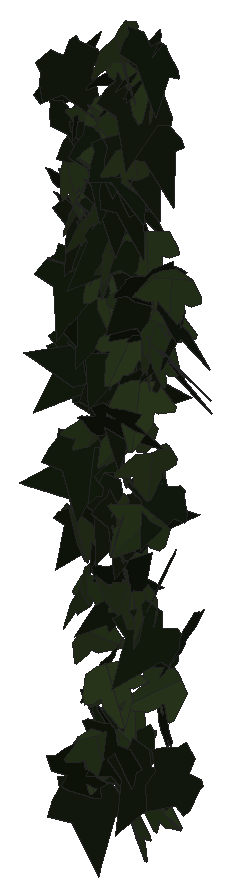
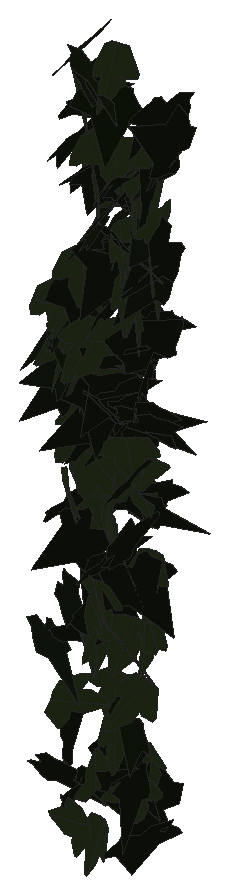
# SketchUp Ruby script. Lengths in inches.
U = 1.inch
M = Sketchup.active_model
def pt(a) = Geom::Point3d.new(a.map { |v| v * U })
def face(e, loops, mat)
  f = e.add_face(loops[0].map { |a| pt(a) })
  loops[1..].each { |l| e.add_face(l.map { |a| pt(a) }).erase! }
  f.material = f.back_material = mat if mat
  f
end
# faces: each face lists its corners as indices into pts; further lists are holes
def faces(e, pts, list, mat = nil) = list.each { |f| face(e, (f[0].is_a?(Array) ? f : [f]).map { |l| l.map { |i| pts[i] } }, mat) }
# xy, xz, yz: faces in a plane at the given z, y or x. An outline is a flat list of corners, or four numbers for a rectangle; further outlines are holes
def ring(l) = l.size == 4 ? [[l[0], l[1]], [l[2], l[1]], [l[2], l[3]], [l[0], l[3]]] : l.each_slice(2).to_a
def flat(e, list, mat, &to3) = list.each { |f| face(e, (f[0].is_a?(Array) ? f : [f]).map { |l| ring(l).map { |u, v| to3.(u, v) } }, mat) }
def xy(e, z, list, mat = nil) = flat(e, list, mat) { |x, y| [x, y, z] }
def xz(e, y, list, mat = nil) = flat(e, list, mat) { |x, z| [x, y, z] }
def yz(e, x, list, mat = nil) = flat(e, list, mat) { |y, z| [x, y, z] }
def lines(e, pts, list) = list.each { |a, b| e.add_line(pt(pts[a]), pt(pts[b])) }
# prism: a flat outline (further loops are holes) pulled along v
def prism(e, loops, v, mat = nil)
  f = face(e, loops, mat); d = Geom::Vector3d.new(v.map { |x| x * U })
  f.pushpull(f.normal.samedirection?(d) ? d.length : -d.length)
end
def box(e, o, s, mat = nil) = prism(e, [[o, [o[0] + s[0], o[1], o[2]], [o[0] + s[0], o[1] + s[1], o[2]], [o[0], o[1] + s[1], o[2]]]], [0, 0, s[2]], mat)
def at(x, y, z, deg = 0) = Geom::Transformation.translation(pt([x, y, z])) * Geom::Transformation.rotation(ORIGIN, Z_AXIS, deg.degrees)
def axes(o, x, y, z) = Geom::Transformation.new([*x, 0, *y, 0, *z, 0, *pt(o).to_a, 1])
def part(name) = M.definitions.add(name)
# library, detail: a bought-in or finely detailed component or shape, given as its bounding box
def library(name, o, s) = part(name).tap { |d| box(d.entities, o, s) }
def detail(e, o, s) = box(e.add_group.entities, o, s)
def put(e, d, t, mat = nil) = e.add_instance(d, t).tap { |i| i.material = mat if mat }
def group(e, t, mat = nil) = e.add_group.tap { |g| g.transformation = t; g.material = mat if mat }.entities
root = M.entities
M.materials.add("efeu1").color = [18, 25, 13]
M.materials.add("efeu2").color = [43, 57, 29]
c1 = part("ivyleaf_9")
p = [[1.54,2.16,1.25],[1.36,2.04,1.19],[-0.21,0.99,0.68],[-0.71,1.11,0.82],[-0.85,0.86,0.67],[-0.8,0.17,0.21],
  [-0.9,-0.01,0.1],[-0.67,-0.16,-0.02],[-0.08,-0.08,-0.05],[-0.03,-0.6,-0.4],[0.65,-0.88,-0.66],[0.83,-0.6,-0.49],
  [1.29,-0.42,-0.43],[1.8125,-0.07,-0.26],[1.21,0.44,0.15]]
faces(c1.entities,p,[[0,1,2,3,4,5,6,7,8,9,10,11,12,13,14]],"efeu1")
c2 = part("ivyleaf_10")
p = [[0,0.5,-0.03],[-0.0625,2.02,-0.43],[-0.19,2.01,-0.46],[-0.54,1.05,-0.29],[-0.52,0.625,-0.18],[-0.83,0.76,-0.28],
  [-1.16,0.64,-0.33],[-1.15,0.33,-0.24],[-0.77,-0.39,0.02],[-0.3,-0.51,0.16],[0.04,-0.48,0.23],[-0.02,2.01,-0.4375],
  [-0.06,2.01,-0.43],[0.04,-0.49,0.23],[0.67,-0.49,0.14],[1.38,0.36,-0.2],[1.375,0.51,-0.24],[0.81,0.65,-0.19],
  [0.62,0.59,-0.15],[0.6,1.09,-0.28],[0.5,1.23,-0.31]]
faces(c2.entities,p,[[0,1,2,3,4,5,6,7,8,9,10],[11,12,0,13,14,15,16,17,18,19,20]],"efeu2")
put(root,c1,axes([555.37,131.1,236.45],[0.02689,-0.13384,0.95916],[0.62063,0.73899,0.08572],[-0.74346,0.61205,0.10625]))
put(root,c1,axes([555.43,131.6,232.75],[0.95601,0.10212,-0.10441],[-0.1051,0.00093,-0.96137],[-0.10142,0.96169,0.01202]))
put(root,c2,axes([555.83,131.82,231.69],[0.41811,-0.87537,-0.0637],[0.06127,0.0995,-0.96514],[0.87555,0.41107,0.09797]))
put(root,c1,axes([556.1875,132.05,225.11],[-0.8463,-0.33405,0.13391],[-0.10601,-0.09561,-0.9085],[0.34393,-0.85148,0.04948]))
put(root,c1,axes([556.11,132.44,225.83],[-0.7996,-0.47085,-0.07469],[0.06122,0.04323,-0.92791],[0.47279,-0.80191,-0.00616]))
put(root,c1,axes([555.62,131.73,231.7],[0.94441,0.04045,-0.16656],[-0.16916,0.0696,-0.94224],[-0.02763,0.95645,0.07561]))
put(root,c1,axes([556.18,131.64,234.32],[0.02952,-0.38642,0.96852],[0.17134,0.95754,0.37682],[-1.02859,0.14841,0.09056]))
put(root,c1,axes([556.8,132.03,224.96],[-0.44942,0.0005,0.89544],[-0.89541,0.00788,-0.44941],[-0.00727,-1.00186,-0.00308]))
put(root,c1,axes([556.28,132.41,210.52],[0.68966,0.055,-0.739],[-0.74058,0.01515,-0.69],[-0.02643,1.01071,0.05055]))
put(root,c2,axes([556.1,131.22,233.5],[-0.08963,0.96019,0.05758],[-0.04433,0.05364,-0.96357],[-0.96089,-0.09204,0.03908]))
put(root,c1,axes([556.53,132.11,218.81],[0.18482,0.5254,-0.84591],[-0.2453,-0.80982,-0.55658],[-0.9651,0.30645,-0.02053]))
put(root,c2,axes([556.34,131.32,218.85],[-0.89072,0.24427,0.11586],[-0.11013,0.0365,-0.92359],[-0.24691,-0.89748,-0.00603]))
put(root,c1,axes([556.92,131.26,220.96],[-0.73932,0.08568,0.56516],[-0.56781,-0.00366,-0.74224],[-0.06584,-0.93058,0.05495]))
put(root,c1,axes([555.93,131.05,238.15],[0.17485,-0.71635,-0.68512],[-0.1145,0.67644,-0.7365],[0.9846,0.20588,0.03602]))
put(root,c1,axes([556.24,131.6,229.28],[-0.66043,-0.65762,-0.18862],[0.14763,0.11899,-0.9318],[0.66801,-0.67645,0.01946]))
put(root,c1,axes([555.76,132.01,228.4],[1.03081,0.17194,0.04386],[-0.04432,-0.00091,1.04503],[0.17182,-1.03174,0.00639]))
put(root,c1,axes([555.95,133.19,223.28],[0.14447,-0.90416,0.10259],[0.01665,-0.10123,-0.91563],[0.90981,0.14543,0.00047]))
put(root,c2,axes([556.2,132.81,224.5],[0.80714,0.45763,-0.05627],[-0.0491,-0.0275,-0.92785],[-0.45846,0.80863,0.00029]))
put(root,c1,axes([555.76,131.59,235.57],[0.36085,-0.89036,0.19543],[0.20608,-0.12506,-0.95029],[0.88796,0.39086,0.14113]))
put(root,c1,axes([556.51,133.11,220.03],[-0.22171,-0.14264,0.88694],[-0.4483,-0.77409,-0.23656],[0.77848,-0.4864,0.11637]))
put(root,c1,axes([556.67,131.01,232.82],[0.00508,0.63079,0.83793],[0.01187,0.83785,-0.6308],[-1.04875,0.01254,-0.00308]))
put(root,c2,axes([556.55,131.09,216.12],[0.07164,-0.73017,-0.69798],[-0.07508,0.69395,-0.73366],[1.00732,0.10365,-0.00504]))
put(root,c2,axes([556.26,132.09,213.88],[-0.25192,-0.54666,-0.73995],[0.35186,0.65161,-0.60119],[0.85003,-0.43174,0.02956]))
put(root,c1,axes([556.26,132.14,231.06],[-0.25038,-0.80938,0.46528],[0.00867,-0.48372,-0.83679],[0.93354,-0.21258,0.13256]))
put(root,c1,axes([556.16,132.15,226.375],[0.33959,-0.73444,-0.50214],[0.51009,-0.27964,0.75397],[-0.72894,-0.53784,0.29368]))
put(root,c1,axes([556.85,131.86,212.31],[-0.15047,0.76761,0.52063],[-0.08965,0.51293,-0.78217],[-0.92317,-0.17493,-0.00891]))
put(root,c2,axes([556.51,131.97,229.97],[0.59829,-0.73894,-0.21917],[-0.00107,0.27665,-0.93568],[0.77076,0.57398,0.16883]))
put(root,c2,axes([556.72,131.83,222.77],[-0.31262,-0.83811,0.26236],[-0.09271,-0.24543,-0.89451],[0.8733,-0.32608,-0.00105]))
put(root,c2,axes([556.61,132.43,230.98],[0.00044,-0.93504,-0.1991],[0.04483,0.1989,-0.93401],[0.95495,-0.00891,0.04394]))
put(root,c1,axes([556.45,131.5625,221.89],[-0.36618,-0.84517,-0.20789],[0.08134,0.19133,-0.92108],[0.86655,-0.37511,-0.00139]))
put(root,c2,axes([556.66,131.73,233.89],[0.34195,-0.90255,-0.20089],[-0.0009,0.21386,-0.96236],[0.92463,0.33399,0.07335]))
put(root,c1,axes([556.43,132.61,219.1],[-0.5592,0.00614,-0.72735],[0.71672,-0.1518,-0.55231],[-0.12404,-0.90482,0.08772]))
put(root,c2,axes([557.1,131.57,235.76],[-0.87232,-0.29938,0.29897],[-0.27884,-0.10846,-0.9222],[0.31821,-0.91574,0.01148]))
put(root,c1,axes([556.77,132.34,227.85],[-0.58465,-0.7611,-0.0035],[0.09169,-0.06604,-0.95306],[0.75557,-0.58092,0.11294]))
put(root,c1,axes([556.52,131.73,207.46],[-0.12604,-1.01416,-0.28006],[0.09635,0.26975,-1.02019],[1.04769,-0.14681,0.06013]))
put(root,c2,axes([556.74,131.82,209.4],[0.65969,0.57269,-0.04042],[-0.03054,-0.02648,-0.8736],[-0.57331,0.6604,0.00002]))
put(root,c2,axes([556.87,131.97,216.18],[-0.82623,-0.33268,-0.21949],[0.19686,0.09862,-0.89052],[0.34655,-0.84918,-0.01743]))
put(root,c1,axes([557.72,131.77,232.06],[-0.54638,0.47653,0.63127],[-0.52747,0.35218,-0.7224],[-0.58937,-0.75697,0.0613]))
put(root,c2,axes([557,131.8125,231.49],[0.24326,-0.88016,-0.33975],[0.05396,0.36327,-0.90244],[0.94191,0.2065,0.13944]))
put(root,c1,axes([556.27,130.92,208.41],[0.34963,0.01544,0.92468],[0.92348,0.04718,-0.34996],[-0.04959,0.98744,0.00227]))
put(root,c2,axes([557.15,130.87,231.93],[0.03796,-0.90385,-0.38317],[0.01737,0.38401,-0.90412],[0.98156,0.02816,0.03082]))
put(root,c1,axes([557.13,132.35,226.26],[-0.41627,-0.8496,0.05665],[-0.01456,-0.05594,-0.94602],[0.85136,-0.41636,0.01152]))
put(root,c2,axes([557.3125,132.17,212.13],[-0.10485,-0.88455,-0.2076],[0.0422,0.20401,-0.89057],[0.9076,-0.11168,0.01742]))
put(root,c1,axes([557,131.64,234.95],[-0.19642,-0.93581,-0.22969],[0.06542,0.22092,-0.95603],[0.96137,-0.20623,0.01813]))
put(root,c1,axes([557.72,131.97,215.96],[-0.84974,0.41026,-0.04875],[0.04345,-0.02213,-0.94359],[-0.41085,-0.85085,0.00103]))
put(root,c2,axes([557.13,132.03,228.97],[0.40989,0.86251,-0.02569],[-0.01207,-0.02271,-0.95495],[-0.8628,0.41007,0.00116]))
put(root,c2,axes([557.4375,131.65,232.45],[0.05668,-0.97046,-0.11411],[-0.02143,0.11304,-0.972],[0.97691,0.05879,-0.0147]))
put(root,c1,axes([557.27,132.65,219.58],[-0.36141,-0.85485,0.15106],[-0.03543,-0.14896,-0.92778],[0.86738,-0.36228,0.02504]))
put(root,c2,axes([557.42,132.08,236.26],[0.67745,0.69462,-0.04585],[-0.13272,0.06607,-0.95997],[-0.68336,0.67578,0.14099]))
put(root,c2,axes([557.58,130.92,210.1875],[-0.58883,-0.73215,-0.18983],[0.12308,0.14462,-0.93954],[0.74628,-0.60154,0.00517]))
put(root,c1,axes([557.83,132.06,231.84],[-0.80782,-0.49938,0.1584],[-0.1093,-0.12406,-0.94853],[0.51237,-0.8138,0.0474]))
put(root,c1,axes([557.47,131.75,226.53],[0.52794,0.75081,0.22186],[0.09468,0.20439,-0.91702],[-0.77716,0.53494,0.03899]))
put(root,c2,axes([557.1,130.92,209.91],[-0.57511,-0.04177,-0.72546],[0.71937,0.09804,-0.57593],[0.10271,-0.92056,-0.02842]))
put(root,c1,axes([557.24,132.37,224.3],[0.08937,-1.07301,0.08296],[0.01113,-0.08232,-1.07672],[1.07616,0.08996,0.00425]))
put(root,c1,axes([558.27,132.12,209.13],[-0.84316,-0.36222,-0.24054],[-0.20429,-0.13328,0.91678],[-0.38383,0.86662,0.04045]))
put(root,c1,axes([557.78,132.25,226.32],[0.39759,0.83244,-0.21397],[-0.12073,-0.17933,-0.922],[-0.85097,0.41437,0.03083]))
put(root,c1,axes([558.28,131.01,210.27],[0.21497,0.13655,-1.04401],[-0.91033,-0.51132,-0.25432],[-0.52907,0.93527,0.01339]))
put(root,c1,axes([557.42,131.68,234.67],[-0.10943,-0.97813,0.07502],[-0.00037,-0.07545,-0.9842],[0.981,-0.10914,0.008]))
put(root,c1,axes([557.64,131.6875,231.49],[0.4869,0.817,0.23185],[0.07638,0.22405,-0.94989],[-0.84582,0.49055,0.04769]))
put(root,c2,axes([557.63,132.83,218.04],[0.86608,-0.24935,-0.03911],[-0.03626,0.0154,-0.90125],[0.24978,0.86682,0.00476]))
put(root,c1,axes([557.98,131.55,238.1],[0.23705,0.94658,0.0071],[-0.15645,0.0464,-0.96209],[-0.93358,0.23257,0.16303]))
put(root,c2,axes([558.13,132.36,222.94],[-0.44824,-0.6664,0.65634],[-0.33743,-0.56359,-0.80268],[0.87235,-0.56041,0.02677]))
put(root,c1,axes([557.6,132.69,219.03],[-0.13623,-0.89265,0.25627],[0.02598,-0.26258,-0.9008],[0.92835,-0.12364,0.06282]))
put(root,c2,axes([557.74,132.94,217.34],[0.15481,-0.78586,0.41306],[0.23073,-0.36928,-0.78902],[0.85729,0.24129,0.13777]))
put(root,c2,axes([557.43,130.61,234.48],[-0.59104,-0.30552,-0.7503],[0.69421,0.28772,-0.66401],[0.41757,-0.91076,0.04193]))
put(root,c2,axes([557.75,132.65,215.86],[-0.04742,-0.87433,0.09197],[0.31861,-0.10293,-0.81428],[0.81939,-0.01058,0.32195]))
put(root,c2,axes([557.99,132.21,226.62],[0.65257,0.57554,-0.37706],[-0.29475,-0.23575,-0.86996],[-0.62173,0.71586,0.01666]))
put(root,c2,axes([558.29,131.42,221.94],[-0.64742,0.41756,0.57915],[-0.47062,0.33834,-0.77004],[-0.53692,-0.80005,-0.02339]))
put(root,c2,axes([558.01,132.43,209.49],[0.10325,0.88613,-0.27267],[0.03354,0.27061,0.89213],[0.92653,-0.10855,-0.00191]))
put(root,c1,axes([558.19,131.49,231.25],[-0.72877,-0.55795,0.26405],[-0.13803,-0.25088,-0.91111],[0.60164,-0.7334,0.1108]))
put(root,c2,axes([558.07,131.36,230.68],[0.24632,-0.93465,0.15357],[0.01468,-0.15489,-0.96624],[0.94707,0.2455,-0.02496]))
put(root,c1,axes([557.53,131.98,216.42],[0.85104,0.44597,-0.04084],[0.02214,0.0457,0.96034],[0.44729,-0.8508,0.03017]))
put(root,c2,axes([557.94,131.54,218.59],[-0.51756,0.7016,-0.18904],[0.1273,-0.14095,-0.87165],[-0.71539,-0.53267,-0.01834]))
put(root,c2,axes([558.15,131.22,239.49],[-0.11061,-0.90914,-0.53316],[0.11931,0.52184,-0.91459],[1.04717,-0.15549,0.04789]))
put(root,c1,axes([558.3,132.72,225.72],[-0.88539,-0.12323,-0.29911],[0.2959,0.04381,-0.89392],[0.13076,-0.93352,-0.00246]))
put(root,c1,axes([557.69,131.54,232.85],[0.12965,-0.87065,0.39052],[0.15985,-0.36873,-0.87512],[0.94073,0.18264,0.09488]))
put(root,c2,axes([558.18,130.85,231.21],[0.31565,-0.74545,-0.55087],[0.11202,0.60835,-0.75905],[0.92011,0.18167,0.28139]))
put(root,c2,axes([558.2,131.54,219.82],[0.56772,-0.73605,0.04453],[0.02406,-0.03767,-0.92955],[0.73701,0.56822,-0.00395]))
put(root,c2,axes([557.99,132.39,228.37],[-0.74867,-0.53494,-0.57908],[0.49053,0.30908,-0.9197],[0.61715,-0.8946,0.02852]))
put(root,c1,axes([557.91,132.1,233.21],[0.72524,-0.56517,-0.29595],[-0.16968,0.26106,-0.91434],[0.61499,0.73851,0.09673]))
put(root,c2,axes([558.05,130.89,213.11],[0.73225,0.52314,0.32536],[0.25631,0.20087,-0.89982],[-0.56022,0.77569,0.01359]))
put(root,c1,axes([557.91,130.55,224.08],[0.91751,0.30543,0.28421],[0.26659,0.09896,-0.96697],[-0.32093,0.95541,0.0093]))
put(root,c2,axes([558.4,131.86,207.11],[-0.80346,0.49539,-0.05629],[0.04677,-0.03139,-0.9439],[-0.49637,-0.80482,0.00217]))
put(root,c1,axes([558.3,132.33,228.42],[-0.13047,-0.58301,0.7306],[-0.14285,-0.71658,-0.59733],[0.92372,-0.19316,0.01081]))
put(root,c1,axes([558.03,131.73,233.32],[0.34554,-0.91916,-0.07585],[-0.01332,0.07602,-0.98186],[0.92219,0.3455,0.01424]))
put(root,c1,axes([558.24,131.68,224.67],[0.11434,0.20457,-0.93331],[-0.13286,0.93424,0.18849],[0.94618,0.10647,0.13925]))
put(root,c1,axes([558.27,131.49,235.01],[-0.06439,-0.84508,-0.50202],[0.02345,0.50163,-0.84743],[0.98266,-0.06735,-0.01267]))
put(root,c1,axes([559.15,131.32,238.83],[-0.33757,0.84818,0.36437],[-0.29833,0.26691,-0.89771],[-0.8736,-0.4189,0.16577]))
put(root,c2,axes([558.57,131.88,234.6875],[0.56151,-0.7898,-0.14836],[0.0113,0.18873,-0.96195],[0.80353,0.54926,0.1172]))
put(root,c2,axes([558.89,130.91,238.84],[-0.53194,0.61068,0.57282],[-0.41468,0.39743,-0.80877],[-0.72739,-0.67316,0.04216]))
put(root,c2,axes([558.37,131.02,216.04],[-0.82267,0.13145,0.47615],[0.47289,-0.05766,0.83296],[0.14271,0.94878,-0.01535]))
put(root,c2,axes([559.08,131.01,238.18],[0.72026,-0.18086,-0.65603],[-0.62482,0.2027,-0.74188],[0.26961,0.95293,0.03329]))
put(root,c2,axes([558.92,132.23,215.78],[0.62835,-0.57421,-0.46324],[-0.32419,0.33168,-0.85089],[0.66273,0.70668,0.02297]))
put(root,c2,axes([558.75,132.3,226.66],[-0.30229,0.89132,-0.01357],[-0.1077,-0.05074,-0.93373],[-0.8849,-0.29831,0.11828]))
put(root,c1,axes([559.22,131.54,238.625],[-0.7738,0.53138,-0.28784],[0.15785,-0.27369,-0.9296],[-0.58336,-0.77891,0.13027]))
put(root,c2,axes([558.9375,132.09,231.09],[-0.72722,-0.64057,0.00499],[0.10096,-0.12207,-0.95609],[0.63258,-0.71692,0.15833]))
put(root,c2,axes([558.8125,131.68,224.81],[0.58903,0.82635,-0.14893],[-0.09727,-0.11354,-1.01471],[-0.83401,0.59686,0.01316]))
put(root,c1,axes([559.17,131.68,229.84],[0.21098,0.90775,-0.17965],[-0.05123,-0.17252,-0.93189],[-0.92394,0.21685,0.01064]))
put(root,c2,axes([559.56,131.23,219.94],[-0.65043,-0.42498,0.68169],[-0.53932,-0.41904,-0.77582],[0.59535,-0.8439,0.04195]))
put(root,c1,axes([558.57,131.77,235.05],[0.14634,-0.94407,-0.24076],[0.17101,0.26457,-0.93349],[0.95916,0.09687,0.20317]))
put(root,c1,axes([558.95,132.14,209.03],[-0.26216,-0.9,0.43293],[-0.12078,-0.41575,-0.9374],[0.99138,-0.28864,0.00028]))
put(root,c1,axes([558.97,131.75,219.52],[-0.11012,0.32552,-0.88746],[-0.22217,0.85953,0.34284],[0.9188,0.24685,-0.02347]))
put(root,c2,axes([559.55,132.55,212.57],[0.24731,0.21547,-0.88754],[-0.62053,-0.63504,-0.32708],[-0.67015,0.66754,-0.02467]))
put(root,c2,axes([559.22,130.92,235.36],[-0.3923,-0.87903,-0.171],[0.15153,0.11884,-0.95852],[0.8826,-0.41112,0.08855]))
put(root,c1,axes([559.4,132.54,217.27],[-0.57914,0.47345,-0.48352],[0.38221,-0.29634,-0.74796],[-0.55845,-0.69381,-0.01048]))
put(root,c2,axes([558.85,131.93,215.65],[-0.03544,-0.17673,0.90925],[0.59532,-0.70145,-0.11314],[0.70963,0.57963,0.14032]))
put(root,c1,axes([559.63,132.28,210.74],[0.07146,-0.34285,0.88112],[-0.26362,0.84136,0.34876],[-0.90797,-0.27126,-0.03191]))
put(root,c2,axes([559.05,132.85,221.77],[0.64269,-0.56124,0.32236],[0.24268,-0.21217,-0.85325],[0.6,0.68699,-0.00018]))
put(root,c1,axes([559.17,131.46,237.57],[-0.30438,-0.95298,0.01238],[0.01831,-0.01885,-1.00014],[0.95289,-0.30405,0.02318]))
put(root,c2,axes([558.73,132.54,207.59],[-0.23692,0.06611,-0.90975],[0.79716,-0.44184,-0.23971],[-0.44334,-0.82979,0.05516]))
put(root,c2,axes([559.46,132.12,229.62],[-0.75634,-0.51273,-0.26013],[0.20416,0.16231,-0.91355],[0.53747,-0.78318,-0.01903]))
put(root,c2,axes([559.67,131.51,238.14],[0.6064,-0.69178,-0.3586],[-0.19172,0.30796,-0.9183],[0.75525,0.63362,0.05481]))
put(root,c1,axes([559.7,131.78,215.29],[-0.63534,-0.68062,0.22577],[-0.1616,-0.15798,-0.93102],[0.69864,-0.65549,-0.01003]))
put(root,c1,axes([560,132.22,227.34],[-0.73613,0.55613,-0.23962],[0.18643,-0.15073,-0.92256],[-0.57615,-0.75933,0.00763]))
put(root,c1,axes([559.5,132.42,220.82],[-0.26124,-0.82563,0.29254],[-0.03869,-0.2941,-0.86458],[0.87507,-0.25948,0.04911]))
put(root,c1,axes([559.24,132.52,226.15],[0.91229,-0.24716,-0.00393],[-0.00379,0.00103,-0.94518],[0.24717,0.9123,0]))
put(root,c2,axes([559.9,131.04,222.76],[-0.46242,-0.84291,-0.01694],[-0.00308,0.02101,-0.96134],[0.84308,-0.46226,-0.01281]))
put(root,c2,axes([559.5625,131.94,228.05],[-0.21561,-0.56493,-0.76325],[0.41673,0.64699,-0.5966],[0.85325,-0.45875,0.09851]))
put(root,c2,axes([559.9,131.48,227.18],[-0.34796,0.69214,0.66915],[-0.26771,0.61389,-0.77419],[-0.92474,-0.43816,-0.02766]))
put(root,c2,axes([559.93,132.24,229.41],[-0.72918,-0.6166,0.08605],[0.02007,-0.15573,-0.94586],[0.62225,-0.71753,0.13134]))
put(root,c1,axes([559.46,131.71,236.04],[0.26061,-0.92629,-0.17661],[-0.01183,0.18,-0.96155],[0.9429,0.25827,0.03674]))
put(root,c1,axes([559.43,131.65,239.51],[0.09686,-0.94135,0.27937],[0.15463,-0.26259,-0.93845],[0.96967,0.13591,0.12175]))
put(root,c1,axes([559.21,132.3,226.65],[0.79745,-0.42905,0.25621],[0.25507,-0.06545,-0.9035],[0.42973,0.83504,0.06083]))
put(root,c1,axes([560.53,132.22,214.96],[-0.60026,0.84092,0.03289],[-0.01936,0.02659,-1.03317],[-0.84134,-0.60057,0.00031]))
put(root,c1,axes([559.64,132.33,228.375],[0.78258,-0.46447,-0.25853],[-0.18159,0.19885,-0.90691],[0.49959,0.79983,0.07534]))
put(root,c1,axes([560.56,132.26,209.32],[-0.93302,-0.06272,0.18686],[-0.18518,-0.03072,-0.93496],[0.06751,-0.95105,0.01788]))
